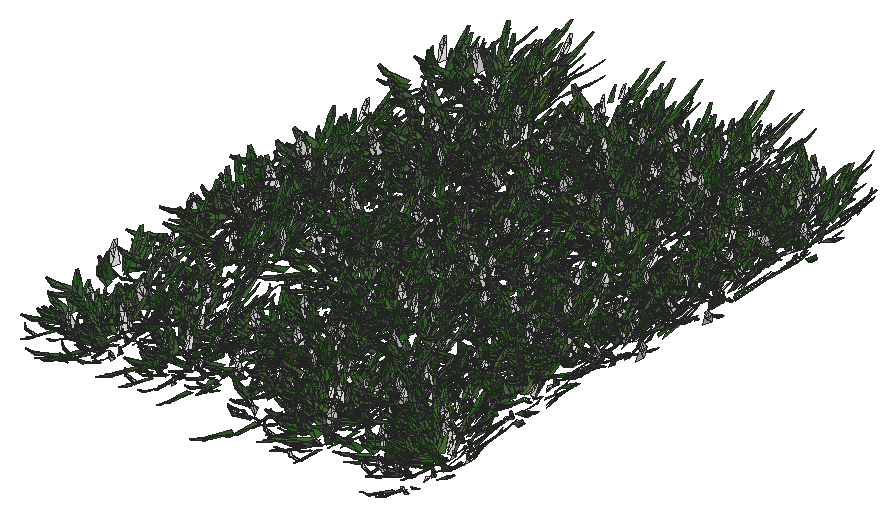
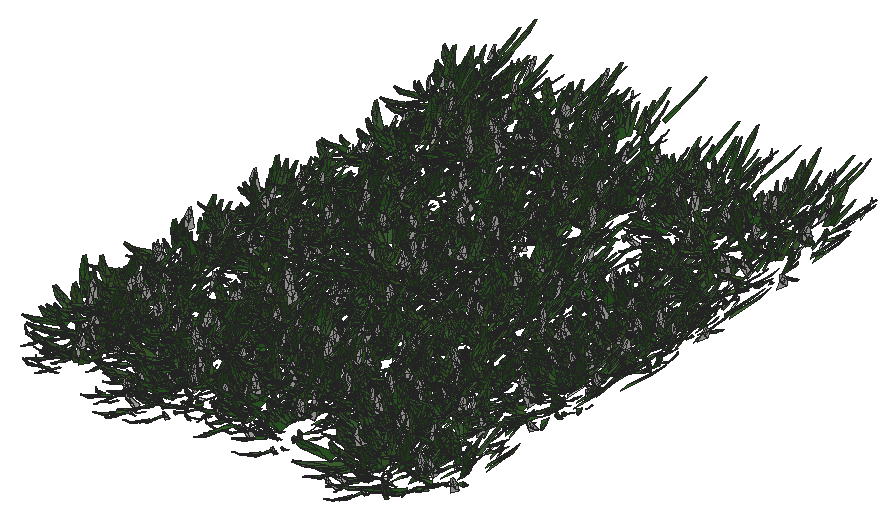
# SketchUp Ruby script. Lengths in inches.
U = 1.inch
M = Sketchup.active_model
def pt(a) = Geom::Point3d.new(a.map { |v| v * U })
def face(e, loops, mat)
  f = e.add_face(loops[0].map { |a| pt(a) })
  loops[1..].each { |l| e.add_face(l.map { |a| pt(a) }).erase! }
  f.material = f.back_material = mat if mat
  f
end
# faces: each face lists its corners as indices into pts; further lists are holes
def faces(e, pts, list, mat = nil) = list.each { |f| face(e, (f[0].is_a?(Array) ? f : [f]).map { |l| l.map { |i| pts[i] } }, mat) }
# xy, xz, yz: faces in a plane at the given z, y or x. An outline is a flat list of corners, or four numbers for a rectangle; further outlines are holes
def ring(l) = l.size == 4 ? [[l[0], l[1]], [l[2], l[1]], [l[2], l[3]], [l[0], l[3]]] : l.each_slice(2).to_a
def flat(e, list, mat, &to3) = list.each { |f| face(e, (f[0].is_a?(Array) ? f : [f]).map { |l| ring(l).map { |u, v| to3.(u, v) } }, mat) }
def xy(e, z, list, mat = nil) = flat(e, list, mat) { |x, y| [x, y, z] }
def xz(e, y, list, mat = nil) = flat(e, list, mat) { |x, z| [x, y, z] }
def yz(e, x, list, mat = nil) = flat(e, list, mat) { |y, z| [x, y, z] }
def lines(e, pts, list) = list.each { |a, b| e.add_line(pt(pts[a]), pt(pts[b])) }
# prism: a flat outline (further loops are holes) pulled along v
def prism(e, loops, v, mat = nil)
  f = face(e, loops, mat); d = Geom::Vector3d.new(v.map { |x| x * U })
  f.pushpull(f.normal.samedirection?(d) ? d.length : -d.length)
end
def box(e, o, s, mat = nil) = prism(e, [[o, [o[0] + s[0], o[1], o[2]], [o[0] + s[0], o[1] + s[1], o[2]], [o[0], o[1] + s[1], o[2]]]], [0, 0, s[2]], mat)
def at(x, y, z, deg = 0) = Geom::Transformation.translation(pt([x, y, z])) * Geom::Transformation.rotation(ORIGIN, Z_AXIS, deg.degrees)
def axes(o, x, y, z) = Geom::Transformation.new([*x, 0, *y, 0, *z, 0, *pt(o).to_a, 1])
def part(name) = M.definitions.add(name)
# library, detail: a bought-in or finely detailed component or shape, given as its bounding box
def library(name, o, s) = part(name).tap { |d| box(d.entities, o, s) }
def detail(e, o, s) = box(e.add_group.entities, o, s)
def put(e, d, t, mat = nil) = e.add_instance(d, t).tap { |i| i.material = mat if mat }
def group(e, t, mat = nil) = e.add_group.tap { |g| g.transformation = t; g.material = mat if mat }.entities
root = M.entities
M.materials.add("Material10").color = [48, 90, 38]
M.materials.add("Material11").color = [68, 110, 48]
M.materials.add("Material12").color = [48, 90, 48]
M.materials.add("Material13").color = [58, 110, 58]
M.materials.add("Material14").color = [58, 90, 38]
M.materials.add("Material15").color = [68, 100, 58]
M.materials.add("Material16").color = [48, 100, 38]
M.materials.add("Material9").color = [68, 110, 58]
c1 = part("grass00")
p = [[-0.6875,0.15,0],[-0.56,0.08,5.52],[-0.04,0.03,2.76],[0.48,-0.02,0],[0.35,-0.02,5.52],[-0.1,-0.14,5.52],
  [-0.12,0.65,8.37],[-0.42,0.65,8.37]]
faces(c1.entities,p,[[0,1,2,3],[3,2,4],[1,5,2],[5,4,2],[1,6,5],[4,5,6],[7,6,1]])
c2 = part("Group16\#1")
put(c2.entities,c1,axes([1.44,-0.61,-0.01],[0.05352,0.12609,0],[-0.10704,0.04543,0.07239],[0.06664,-0.02828,0.11628]),"Material12")
put(c2.entities,c1,axes([0.76,-0.15,-0.01],[0.04676,0.24062,0],[-0.23162,0.04501,0.06642],[0.0652,-0.01267,0.23595]),"Material9")
put(c2.entities,c1,axes([0.79,0.01,-0.01],[-0.00606,0.34651,0],[-0.34381,-0.00602,0.0432],[0.04319,0.00076,0.34386]))
put(c2.entities,c1,axes([1,0.23,-0.01],[-0.07192,0.31144,0],[-0.28722,-0.06632,0.1236],[0.12043,0.02781,0.29478]),"Material11")
put(c2.entities,c1,axes([1.66,0.77,-0.01],[-0.13828,0.29651,0],[-0.21551,-0.1005,0.22471],[0.20365,0.09498,0.23779]),"Material16")
put(c2.entities,c1,axes([0.6875,0.52,-0.01],[-0.18126,0.24051,0],[-0.22746,-0.17142,0.09788],[0.07817,0.05891,0.28481]),"Material11")
put(c2.entities,c1,axes([0.68,0.78,-0.01],[-0.215,0.18688,0],[-0.12385,-0.14248,0.21334],[0.13995,0.16101,0.18878]),"Material9")
put(c2.entities,c1,axes([0.56,1,-0.01],[-0.13756,0.07624,0],[-0.06159,-0.11112,0.0927],[0.04494,0.08108,0.12705]),"Material11")
put(c2.entities,c1,axes([0.2,0.64,-0.01],[-0.23729,0.07254,0],[-0.05711,-0.18681,0.153],[0.04473,0.14632,0.19535]),"Material16")
put(c2.entities,c1,axes([0.0625,0.72,-0.01],[-0.28874,0.02525,0],[-0.02179,-0.24916,0.14647],[0.01276,0.14591,0.25012]),"Material9")
put(c2.entities,c1,axes([-0.08,0.62,-0.01],[-0.34089,-0.04187,0],[0.03255,-0.26504,0.216],[-0.02633,0.21439,0.26703]),"Material16")
put(c2.entities,c1,axes([-0.34,0.98,-0.01],[-0.14314,-0.0493,0],[0.04397,-0.12769,0.06843],[-0.02228,0.0647,0.13505]),"Material16")
put(c2.entities,c1,axes([-0.87,1.45,-0.01],[-0.23488,-0.14114,0],[0.13761,-0.22901,0.06087],[-0.03135,0.05217,0.26717]))
put(c2.entities,c1,axes([-0.72,0.77,-0.01],[-0.14208,-0.13251,0],[0.07209,-0.0773,0.16301],[-0.11118,0.11922,0.1057]),"Material16")
put(c2.entities,c1,axes([-0.62,0.43,-0.01],[-0.14845,-0.21203,0],[0.18654,-0.13061,0.12304],[-0.10079,0.07057,0.22772]),"Material9")
put(c2.entities,c1,axes([-0.68,0.29,-0.01],[-0.13639,-0.32136,0],[0.31723,-0.13464,0.05579],[-0.05136,0.0218,0.34462]),"Material10")
put(c2.entities,c1,axes([-0.64,0.125,-0.01],[-0.0458,-0.23569,0],[0.22124,-0.043,0.08276],[-0.08124,0.01579,0.22538]),"Material13")
put(c2.entities,c1,axes([-1.6,-0.03,-0.01],[0.00576,-0.32897,0],[0.27526,0.00482,0.18018],[-0.18015,-0.00315,0.2753]),"Material11")
put(c2.entities,c1,axes([-1.36,-0.31,-0.01],[0.05718,-0.24765,0],[0.18172,0.04196,0.17267],[-0.16825,-0.03885,0.1865]),"Material16")
put(c2.entities,c1,axes([-1.54,-0.72,-0.01],[0.06537,-0.14017,0],[0.13555,0.06321,0.03939],[-0.0357,-0.01665,0.14956]))
put(c2.entities,c1,axes([-1.19,-0.9,-0.01],[0.09597,-0.12735,0],[0.11214,0.08451,0.07557],[-0.06035,-0.04548,0.14042]),"Material15")
put(c2.entities,c1,axes([-0.47,-0.54,-0.01],[0.11588,-0.10072,0],[0.0618,0.0711,0.12124],[-0.07953,-0.0915,0.0942]))
put(c2.entities,c1,axes([-0.47,-0.84,-0.01],[0.11927,-0.0661,0],[0.06603,0.11913,0.00646],[-0.00313,-0.00565,0.13621]),"Material11")
put(c2.entities,c1,axes([-0.38,-1.24,-0.01],[0.28037,-0.08571,0],[0.0618,0.20215,0.20315],[-0.05939,-0.19428,0.21139]),"Material15")
put(c2.entities,c1,axes([-0.06,-0.66,-0.01],[0.22719,-0.01987,0],[0.01247,0.14255,0.17758],[-0.01547,-0.17691,0.1431]),"Material14")
put(c2.entities,c1,axes([0.11,-0.89,-0.01],[0.14882,0.01828,0],[-0.01058,0.08611,0.12229],[0.01491,-0.12138,0.08676]),"Material12")
put(c2.entities,c1,axes([0.25,-0.72,-0.01],[0.20481,0.07053,0],[-0.06206,0.18022,0.10291],[0.03351,-0.0973,0.1906]),"Material12")
put(c2.entities,c1,axes([0.85,-1.42,-0.01],[0.16481,0.09904,0],[-0.09472,0.15762,0.05616],[0.02893,-0.04814,0.18389]),"Material11")
put(c2.entities,c1,axes([1.01,-1.09,-0.01],[0.21858,0.20385,0],[-0.17495,0.1876,0.15339],[0.10462,-0.11218,0.25652]),"Material16")
put(c2.entities,c1,axes([1.01,-0.71,-0.01],[0.08733,0.12473,0],[-0.06445,0.04512,0.13037],[0.1068,-0.07477,0.07867]),"Material12")
c3 = part("Group15\#1")
put(c3.entities,c2,at(0,0,0))
c4 = part("3darcstudiotree_grass00\#1")
put(c4.entities,c3,at(0,0,0))
put(root,c4,axes([852.99,505.65,12.99],[-1.4574,-5.63848,0],[2.95707,-3.99377,-0.05519],[0.18301,-0.24717,1.81465]))
put(root,c4,axes([868.36,504.57,12.99],[-2.38107,1.42759,0],[-0.85109,-7.41733,-0.03948],[-0.03443,-0.30004,1.58152]))
put(root,c4,axes([880.25,505.71,12.99],[-2.65306,0.75515,0],[-0.30618,-5.6208,-0.03309],[-0.01933,-0.35489,1.60704]))
put(root,c4,axes([812.43,506.21,12.99],[0.97906,6.52331,0],[-3.045,2.38799,-0.02597],[-0.10941,0.0858,1.96681]))
put(root,c4,axes([889.31,505.75,12.99],[-0.29524,7.25073,0],[-3.22684,-0.68655,-0.02425],[-0.09592,-0.02041,1.76617]))
put(root,c4,axes([815.1875,505.93,12.99],[-1.51893,5.13574,0],[-2.21828,-3.42812,-0.04556],[-0.20111,-0.3108,1.95702]))
put(root,c4,axes([864.16,506.36,12.99],[-1.28385,6.32972,0],[-3.05533,-3.23813,-0.04346],[-0.1591,-0.16862,1.86413]))
put(root,c4,axes([829.44,506.47,12.99],[-1.67508,5.71212,0],[-2.30411,-3.53058,-0.02214],[-0.07899,-0.12104,1.63462]))
put(root,c4,axes([860.26,508.67,12.99],[-0.73247,5.58304,0],[-2.39109,-1.63916,-0.04553],[-0.16619,-0.11393,1.30482]))
put(root,c4,axes([804.88,508.77,12.99],[-1.45548,4.78195,0],[-2.53134,-4.02584,-0.02835],[-0.08051,-0.12804,1.46355]))
put(root,c4,axes([836.09,511.61,12.99],[-0.59172,-6.25795,0],[3.15122,-1.55693,-0.06129],[0.18119,-0.08952,1.3376]))
put(root,c4,axes([839.96,513.6,12.99],[1.81889,-5.12817,0],[2.27845,4.22268,-0.02965],[0.0785,0.14549,1.3715]))
put(root,c4,axes([888.95,511.52,12.99],[-2.3306,2.97499,0],[-1.43535,-5.87549,-0.05669],[-0.12758,-0.52224,1.86391]))
put(root,c4,axes([829.74,514.59,12.99],[0.32741,-6.68639,0],[2.88308,0.73767,-0.04376],[0.16602,0.04248,1.51939]))
put(root,c4,axes([813.01,514.53,12.99],[-1.23373,-7.18281,0],[2.85603,-2.56327,-0.05278],[0.2168,-0.19457,1.85719]))
put(root,c4,axes([861.77,514.1,12.99],[3.25038,2.24612,0],[-0.74618,5.64218,-0.04581],[-0.05899,0.44607,1.57403]))
put(root,c4,axes([825.73,515.14,12.99],[-1.6723,-6.27142,0],[2.4813,-3.45726,-0.05337],[0.17283,-0.24081,1.5119]))
put(root,c4,axes([849.57,516.25,12.99],[2.32247,1.67856,0],[-0.87062,6.29427,-0.04459],[-0.05663,0.40941,1.66873]))
put(root,c4,axes([884.89,514.02,12.99],[-2.80487,4.80341,0],[-1.88905,-5.76384,-0.03017],[-0.07229,-0.22059,1.72726]))
put(root,c4,axes([858.34,515.21,12.99],[-1.80171,5.10925,0],[-2.01199,-3.70729,-0.02131],[-0.08871,-0.16345,1.8955]))
put(root,c4,axes([869.47,515.44,12.99],[-3.07015,3.79092,0],[-1.53263,-6.4857,-0.03525],[-0.04956,-0.20972,1.3087]))
put(root,c4,axes([881.875,516.3125,12.99],[-0.66712,7.40109,0],[-2.61738,-1.23277,-0.03296],[-0.12425,-0.05852,1.411]))
put(root,c4,axes([876.95,518.08,12.99],[-1.93115,5.31233,0],[-2.03831,-3.87174,-0.04997],[-0.15521,-0.29482,1.46822]))
put(root,c4,axes([866.54,520.83,12.99],[2.63887,0.34184,0],[-0.16224,6.54434,-0.02759],[-0.00627,0.25286,1.57942]))
put(root,c4,axes([825.33,522.77,12.99],[1.5401,-6.84309,0],[2.33222,2.74265,-0.03693],[0.16201,0.19052,1.77491]))
put(root,c4,axes([870.5,523.34,12.99],[2.02638,-5.28676,0],[2.45049,4.90784,-0.04981],[0.14007,0.28052,1.67091]))
put(root,c4,axes([813.1,521.02,12.99],[-3.22187,-0.62142,0],[0.27101,-7.34215,-0.02802],[0.0096,-0.25998,1.8014]))
put(root,c4,axes([820.1875,522.0625,12.99],[-0.711,6.35229,0],[-2.74123,-1.6032,-0.04208],[-0.16176,-0.09461,1.54007]))
put(root,c4,axes([853.02,523.4375,12.99],[1.90675,3.48333,0],[-1.62246,4.64063,-0.04441],[-0.13783,0.39422,1.772]))
put(root,c4,axes([802.73,524.59,12.99],[2.32676,5.16821,0],[-2.32007,5.45779,-0.06236],[-0.17718,0.41679,1.86199]))
put(root,c4,axes([845.72,524.27,12.99],[-2.90908,1.06809,0],[-0.47179,-6.71432,-0.04907],[-0.03117,-0.44354,1.63442]))
put(root,c4,axes([873.45,524.95,12.99],[-2.41388,2.83907,0],[-1.1343,-5.03934,-0.01759],[-0.04549,-0.2021,1.92222]))
put(root,c4,axes([880.66,527,12.99],[-2.1216,-6.3783,0],[2.389,-4.15221,-0.02],[0.06882,-0.1196,1.779]))
put(root,c4,axes([835.54,526.35,12.99],[-3.3333,-0.68172,0],[0.28526,-7.28818,-0.03473],[0.01209,-0.30896,1.7157]))
put(root,c4,axes([845.32,531.41,12.99],[2.43681,-0.70234,0],[0.39054,7.08027,-0.05027],[0.02289,0.41505,1.55905]))
put(root,c4,axes([880.5,532.96,12.99],[-0.25821,-7.75837,0],[3.42476,-0.59557,-0.05882],[0.1991,-0.03462,1.5994]))
put(root,c4,axes([849.96,530.97,12.99],[-2.90283,-0.7377,0],[0.33963,-6.98326,-0.05312],[0.02325,-0.47813,1.67036]))
put(root,c4,axes([864.83,531.24,12.99],[0.69475,7.78834,0],[-3.04078,1.41733,-0.03996],[-0.13023,0.0607,1.416]))
put(root,c4,axes([816.67,533.64,12.99],[0.37282,-6.86084,0],[2.81263,0.79861,-0.05019],[0.19607,0.05567,1.53052]))
put(root,c4,axes([887.1,532.5,12.99],[0.35558,6.56207,0],[-3.3357,0.94446,-0.03401],[-0.10285,0.02912,1.40523]))
put(root,c4,axes([805.42,536.24,12.99],[1.90294,-4.7288,0],[2.2471,4.72498,-0.05921],[0.19967,0.41984,1.91907]))
put(root,c4,axes([839.71,534.08,12.99],[-2.59691,0.5149,0],[-0.25923,-6.83164,-0.04163],[-0.01656,-0.4363,1.89396]))
put(root,c4,axes([857.34,539.39,12.99],[2.43439,3.40044,0],[-1.76464,6.60107,-0.04231],[-0.09132,0.34162,1.92144]))
put(root,c4,axes([839.84,539.8,12.99],[-1.45752,-6.19148,0],[2.71951,-3.34515,-0.04084],[0.13434,-0.16525,1.58232]))
put(root,c4,axes([860.12,539.4,12.99],[-2.51578,-4.78006,0],[1.576,-4.33412,-0.01701],[0.0629,-0.17297,1.95649]))
put(root,c4,axes([815.08,541,12.99],[2.38977,3.66494,0],[-1.62004,5.51977,-0.0468],[-0.10494,0.35754,1.60535]))
put(root,c4,axes([874.49,542.68,12.99],[1.98103,-6.08526,0],[2.65627,4.51844,-0.05496],[0.13739,0.2337,1.41537]))
put(root,c4,axes([865.81,543.64,12.99],[-3.33016,-0.57714,0],[0.25097,-7.56677,-0.05601],[0.01294,-0.39002,1.39118]))
put(root,c4,axes([846.09,544.49,12.99],[0.0746,5.9936,0],[-3.01911,0.19636,-0.02239],[-0.09931,0.00646,1.83839]))
put(root,c4,axes([850.24,544.17,12.99],[-1.58504,4.29019,0],[-2.2915,-4.42372,-0.03207],[-0.11857,-0.22889,1.99077]))
put(root,c4,axes([876.75,545.08,12.99],[-0.19204,5.84834,0],[-2.72443,-0.46745,-0.02554],[-0.1116,-0.01915,1.64241]))
put(root,c4,axes([885.38,545.98,12.99],[-0.5077,7.35912,0],[-3.20418,-1.15505,-0.03641],[-0.11745,-0.04234,1.45326]))
put(root,c4,axes([852.48,549.64,12.99],[3.15458,-0.54286,0],[0.19816,6.01692,-0.02417],[0.00906,0.27525,1.80918]))
put(root,c4,axes([870.48,548.67,12.99],[1.1771,5.17385,0],[-2.54636,3.02707,-0.03549],[-0.12211,0.14517,1.52707]))
put(root,c4,axes([816.42,550,12.99],[3.02632,-0.99105,0],[0.349,5.56861,-0.032],[0.02684,0.4283,1.99674]))
put(root,c4,axes([840.36,549.01,12.99],[-0.58462,5.91029,0],[-3.36979,-1.7417,-0.04071],[-0.12055,-0.06231,1.43871]))
put(root,c4,axes([801.35,551.99,12.99],[2.11041,6.11928,0],[-2.06545,3.7221,-0.04305],[-0.14239,0.2566,1.51958]))
put(root,c4,axes([833.23,553.14,12.99],[-1.60574,-6.2565,0],[2.52697,-3.38882,-0.03431],[0.11337,-0.15204,1.53951]))
put(root,c4,axes([876.51,551.16,12.99],[-2.25431,2.5457,0],[-1.29842,-6.00796,-0.03032],[-0.05012,-0.23192,1.50108]))
put(root,c4,axes([805.12,550.91,12.99],[-1.92848,6.00161,0],[-2.55415,-4.28843,-0.02364],[-0.08497,-0.14266,1.93862]))
put(root,c4,axes([827.79,552.36,12.99],[-3.03045,-0.65443,0],[0.27243,-6.59187,-0.03137],[0.00982,-0.23769,1.3228]))
put(root,c4,axes([812.43,554.23,12.99],[2.3353,4.92273,0],[-2.21925,5.50107,-0.03053],[-0.09029,0.22382,1.95907]))
put(root,c4,axes([850.375,552.81,12.99],[-2.24312,5.82887,0],[-2.59367,-5.2154,-0.06393],[-0.14229,-0.28613,1.40472]))
put(root,c4,axes([835.83,554.16,12.99],[1.72753,6.45956,0],[-2.20476,3.08098,-0.02868],[-0.10456,0.14612,1.51486]))
put(root,c4,axes([848.46,559.12,12.99],[-1.22805,-6.52328,0],[3.02457,-2.97521,-0.04688],[0.1596,-0.15699,1.67419]))
put(root,c4,axes([868.99,558.25,12.99],[-2.52764,0.67669,0],[-0.29962,-5.84788,-0.03745],[-0.01856,-0.36216,1.50509]))
put(root,c4,axes([828.84,559.06,12.99],[-2.12795,-3.77701,0],[2.07578,-6.11082,-0.06125],[0.1101,-0.32411,1.36064]))
put(root,c4,axes([872.72,560.9375,12.99],[3.30833,0.81692,0],[-0.37386,7.91113,-0.03307],[-0.01185,0.2508,1.59331]))
put(root,c4,axes([845.09,560.16,12.99],[-1.95649,-5.83038,0],[2.26162,-3.96557,-0.03114],[0.1185,-0.20778,1.87535]))
put(root,c4,axes([823.93,559.13,12.99],[-3.32319,-1.70739,0],[0.6152,-6.2567,-0.03373],[0.02563,-0.26063,1.33323]))
put(root,c4,axes([889.4,561.07,12.99],[-1.7474,-5.59847,0],[2.13202,-3.47712,-0.04134],[0.18201,-0.29685,1.943]))
put(root,c4,axes([882.71,560.52,12.99],[-2.64394,-4.70193,0],[2.10499,-6.18488,-0.06227],[0.11154,-0.32773,1.37168]))
put(root,c4,axes([860.16,562.42,12.99],[1.4135,-7.23952,0],[2.95986,3.0197,-0.04062],[0.14934,0.15236,1.79015]))
put(root,c4,axes([886.85,561.05,12.99],[2.07856,3.7481,0],[-2.10175,6.0903,-0.06164],[-0.11086,0.32125,1.3518]))
put(root,c4,axes([865.9,561.49,12.99],[-2.25962,-5.14073,0],[2.21805,-5.09433,-0.05331],[0.14975,-0.34394,1.71744]))
put(root,c4,axes([832.41,563.39,12.99],[1.66204,-4.39015,0],[2.41371,4.77477,-0.03846],[0.1049,0.2075,1.57923]))
put(root,c4,axes([800.16,561.98,12.99],[-2.26266,-2.51888,0],[1.23228,-5.78396,-0.03924],[0.0859,-0.40317,1.93013]))
put(root,c4,axes([807.05,562.32,12.99],[-3.24556,-2.91538,0],[1.09584,-6.37452,-0.03326],[0.04569,-0.26579,1.54402]))
put(root,c4,axes([858.6,563.05,12.99],[-3.20164,0.80461,0],[-0.27498,-5.71731,-0.04038],[-0.0204,-0.42407,1.5952]))
put(root,c4,axes([877.9,563.14,12.99],[-1.08518,6.28319,0],[-3.06147,-2.76285,-0.02576],[-0.0813,-0.07337,1.53201]))
put(root,c4,axes([852.31,563.375,12.99],[-2.65665,4.62743,0],[-1.7035,-5.11023,-0.04347],[-0.11366,-0.34096,1.66314]))
put(root,c4,axes([803.65,563.48,12.99],[-2.01396,5.33847,0],[-2.62607,-5.17661,-0.04683],[-0.13903,-0.27406,1.86493]))
put(root,c4,axes([809.43,567.39,12.99],[2.31786,-4.07708,0],[1.57903,4.69065,-0.03629],[0.08811,0.26173,1.41389]))
put(root,c4,axes([850.25,568.15,12.99],[3.37025,-0.741,0],[0.33309,7.91597,-0.06081],[0.01765,0.4194,1.44654]))
put(root,c4,axes([873.7,568.48,12.99],[1.82139,-5.98472,0],[2.10675,3.35024,-0.02795],[0.12137,0.19301,1.86246]))
put(root,c4,axes([812.13,569.21,12.99],[2.70657,0.01219,0],[-0.0049,5.68045,-0.0306],[-0.00034,0.39037,1.9022]))
put(root,c4,axes([840.26,569.43,12.99],[2.23742,2.46538,0],[-1.09622,5.19834,-0.04063],[-0.07804,0.37007,1.53169]))
put(root,c4,axes([823.875,568.59,12.99],[-3.45981,1.22272,0],[-0.39983,-5.91155,-0.03554],[-0.02778,-0.41075,1.83631]))
put(root,c4,axes([804.48,571.53,12.99],[0.52589,-5.69614,0],[3.19216,1.53995,-0.04294],[0.126,0.06079,1.34209]))
put(root,c4,axes([856.76,571.46,12.99],[-0.35187,-6.78121,0],[3.07514,-0.83377,-0.02638],[0.08909,-0.02416,1.44452]))
put(root,c4,axes([869.74,569.67,12.99],[0.65067,6.54246,0],[-3.24751,1.68762,-0.06457],[-0.19925,0.10354,1.44574]))
put(root,c4,axes([829.5,571.44,12.99],[-1.60291,-6.07943,0],[2.15074,-2.96305,-0.03107],[0.12859,-0.17716,1.66455]))
put(root,c4,axes([860.02,572.91,12.99],[1.13793,-5.04136,0],[2.78043,3.27934,-0.04957],[0.1772,0.20899,1.72633]))
put(root,c4,axes([885.14,571.39,12.99],[-2.7214,-1.55169,0],[0.64329,-5.89517,-0.04204],[0.04537,-0.41582,1.62585]))
put(root,c4,axes([814.9375,573.63,12.99],[2.65986,-1.80196,0],[0.71387,5.506,-0.03127],[0.03837,0.29597,1.48816]))
put(root,c4,axes([844.01,572.72,12.99],[1.01083,5.48152,0],[-2.89471,2.78925,-0.04214],[-0.17447,0.16812,1.93625]))
put(root,c4,axes([803.75,578.67,12.99],[1.55106,-4.40014,0],[2.61135,4.80987,-0.04335],[0.11342,0.2089,1.54559]))
put(root,c4,axes([873.3,578.83,12.99],[1.85863,-5.65045,0],[2.79417,4.8025,-0.05965],[0.1964,0.33757,1.97549]))
put(root,c4,axes([833.6875,576.82,12.99],[-2.58612,-2.20778,0],[1.17469,-7.18988,-0.03885],[0.05262,-0.32206,1.78292]))
put(root,c4,axes([877.1875,579.49,12.99],[3.08374,-0.337,0],[0.11769,5.62734,-0.03217],[0.00788,0.37663,1.73328]))
put(root,c4,axes([828.51,580.52,12.99],[0.08733,-7.9419,0],[2.89886,0.16655,-0.05528],[0.22204,0.01276,1.59813]))
put(root,c4,axes([849.59,579.93,12.99],[-1.15076,-7.02922,0],[3.20384,-2.74064,-0.05081],[0.15149,-0.12959,1.49393]))
put(root,c4,axes([845.95,581.6875,12.99],[2.16351,-3.14925,0],[1.41509,5.07972,-0.0345],[0.09485,0.34047,1.8497]))
put(root,c4,axes([885.41,579.84,12.99],[0.1113,5.63218,0],[-2.73633,0.28256,-0.0329],[-0.17342,0.01791,1.98251]))
put(root,c4,axes([890.27,581.6875,12.99],[-2.23602,-4.99913,0],[2.07036,-4.83873,-0.0483],[0.13186,-0.30816,1.58573]))
put(root,c4,axes([809.34,581.74,12.99],[-2.91102,-3.24885,0],[1.51961,-7.11461,-0.06565],[0.1031,-0.48269,1.70067]))
put(root,c4,axes([820.73,583.67,12.99],[-0.54687,-6.17378,0],[2.7682,-1.28126,-0.04711],[0.1797,-0.08317,1.50792]))
put(root,c4,axes([801.32,581.74,12.99],[-2.98379,-0.69531,0],[0.32782,-7.35077,-0.03002],[0.01098,-0.24613,1.59842]))
put(root,c4,axes([828.12,586.77,12.99],[-1.12297,-6.7513,0],[3.24762,-2.82262,-0.02869],[0.07921,-0.06884,1.40786]))
put(root,c4,axes([836.04,587.03,12.99],[-0.95373,-6.80216,0],[2.91754,-2.13748,-0.03893],[0.14493,-0.10618,1.64312]))
put(root,c4,axes([883.01,588.375,12.99],[2.8313,4.41831,0],[-1.6421,5.49838,-0.02215],[-0.05923,0.19831,1.8946]))
put(root,c4,axes([865.1,589.73,12.99],[1.78996,-5.10233,0],[2.42773,4.4502,-0.04277],[0.12531,0.22971,1.60323]))
put(root,c4,axes([803.27,589.24,12.99],[2.78821,2.27626,0],[-1.15946,7.42104,-0.02984],[-0.033,0.21122,1.55474]))
put(root,c4,axes([851.99,588.33,12.99],[-2.77583,-4.90355,0],[1.98262,-5.86445,-0.06061],[0.11968,-0.354,1.43628]))
put(root,c4,axes([820.84,589.99,12.99],[2.73638,0.13485,0],[-0.05769,6.11729,-0.0399],[-0.00442,0.46833,1.8861]))
put(root,c4,axes([841.42,590.68,12.99],[2.71897,0.8946,0],[-0.4236,6.72716,-0.04848],[-0.02557,0.40614,1.51023]))
put(root,c4,axes([888.82,590.3,12.99],[3.03645,1.93549,0],[-0.7103,5.82269,-0.03867],[-0.05028,0.41218,1.75619]))
put(root,c4,axes([860.07,591.58,12.99],[2.32563,-1.97622,0],[1.0064,6.18842,-0.02775],[0.04696,0.28874,1.92398]))
put(root,c4,axes([812.02,589.67,12.99],[-3.07362,-0.06655,0],[0.03292,-7.94545,-0.04475],[0.00127,-0.30764,1.43393]))
put(root,c4,axes([867.98,591.37,12.99],[-2.94786,3.38613,0],[-1.22018,-5.55051,-0.0516],[-0.12101,-0.55045,1.94674]))
put(root,c4,axes([843.88,591.9,12.99],[-1.50123,6.04582,0],[-2.93059,-3.80236,-0.03094],[-0.07874,-0.10216,1.35284]))
put(root,c4,axes([843.74,597.46,12.99],[2.93963,-0.43219,0],[0.216,7.67669,-0.04097],[0.00947,0.33665,1.66267]))
put(root,c4,axes([860.38,595.68,12.99],[-2.62956,-1.70091,0],[0.67288,-5.43554,-0.03071],[0.03421,-0.27638,1.38702]))
put(root,c4,axes([866,598.39,12.99],[3.24457,-1.97014,0],[0.87275,7.51027,-0.06211],[0.05478,0.47139,1.60192]))
put(root,c4,axes([822.9375,596.34,12.99],[-0.07625,6.66774,0],[-3.02885,-0.18099,-0.03889],[-0.14122,-0.00844,1.50954]))
put(root,c4,axes([821.27,598.71,12.99],[-0.23839,-5.75072,0],[3.38736,-0.73373,-0.03587],[0.12273,-0.02658,1.60406]))
put(root,c4,axes([836.24,598.65,12.99],[-2.49285,-5.43926,0],[2.26095,-5.41443,-0.04863],[0.14628,-0.35031,1.95701]))
put(root,c4,axes([853.67,597.36,12.99],[-2.9804,0.5478,0],[-0.25056,-7.12315,-0.04274],[-0.01047,-0.29752,1.31001]))
put(root,c4,axes([815.39,597.57,12.99],[-2.5937,4.97056,0],[-1.98974,-5.42522,-0.04843],[-0.10388,-0.28325,1.41858]))
put(root,c4,axes([868.73,599.66,12.99],[3.09205,3.53048,0],[-1.38455,6.33616,-0.04234],[-0.0639,0.29243,1.4356]))
put(root,c4,axes([856.2,600.94,12.99],[2.81397,-2.72741,0],[1.13396,6.11325,-0.02583],[0.04269,0.23015,1.68703]))
put(root,c4,axes([881.99,598.36,12.99],[-1.1808,6.41553,0],[-2.38617,-2.29484,-0.02216],[-0.09563,-0.09197,1.66252]))
put(root,c4,axes([847.65,601.23,12.99],[-1.94835,-5.48536,0],[2.6094,-4.84293,-0.02494],[0.08226,-0.15266,1.95866]))
put(root,c4,axes([827.9,600.88,12.99],[-1.22338,5.27333,0],[-2.21347,-2.68322,-0.02105],[-0.10183,-0.12344,1.88169]))
put(root,c4,axes([825.39,606.4,12.99],[1.55699,-6.71187,0],[3.01256,3.65161,-0.05067],[0.14506,0.17584,1.51576]))
put(root,c4,axes([839.37,604.98,12.99],[-2.63123,-4.92353,0],[1.78386,-4.98135,-0.04086],[0.1178,-0.32894,1.75811]))
put(root,c4,axes([820.36,606.5625,12.99],[1.83456,-4.46525,0],[2.03909,4.37751,-0.02466],[0.07472,0.1604,1.59511]))
put(root,c4,axes([885.32,606.97,12.99],[2.44886,-2.36198,0],[1.33512,7.23289,-0.0407],[0.05083,0.27539,1.51351]))
put(root,c4,axes([832.73,607.58,12.99],[1.94903,-6.24142,0],[2.70718,4.41731,-0.04124],[0.11484,0.18738,1.56101]))
put(root,c4,axes([888.9375,604.87,12.99],[-2.7025,0.34216,0],[-0.16171,-6.674,-0.04105],[-0.01037,-0.42804,1.83253]))
put(root,c4,axes([811.67,607.23,12.99],[0.05202,-7.34397,0],[3.47529,0.12862,-0.02796],[0.09347,0.00346,1.59394]))
put(root,c4,axes([852.65,606.07,12.99],[1.85754,4.66138,0],[-2.41325,5.02493,-0.05824],[-0.15142,0.3153,1.57486]))
put(root,c4,axes([879.04,604.92,12.99],[-1.70476,5.28626,0],[-2.10539,-3.54773,-0.0238],[-0.08539,-0.14389,1.59896]))
put(root,c4,axes([827.93,605.4,12.99],[-1.25637,6.42574,0],[-2.40386,-2.45588,-0.0353],[-0.15984,-0.16329,1.79152]))
put(root,c4,axes([866.23,607.53,12.99],[3.08918,3.63476,0],[-1.49736,6.64962,-0.04224],[-0.06825,0.30308,1.58426]))
put(root,c4,axes([881.64,609.29,12.99],[2.48701,-4.31869,0],[1.62379,4.88608,-0.03309],[0.07839,0.23589,1.44206]))
put(root,c4,axes([868.37,608.19,12.99],[-2.8365,0.59895,0],[-0.23568,-5.83204,-0.04806],[-0.01996,-0.49394,1.58689]))
put(root,c4,axes([804.93,610.5,12.99],[0.83911,-5.72905,0],[3.01878,2.31034,-0.04023],[0.11918,0.09121,1.36415]))
put(root,c4,axes([856.24,608.28,12.99],[-1.23548,5.6059,0],[-2.55924,-2.94719,-0.03585],[-0.1292,-0.14878,1.58646]))
put(root,c4,axes([816.15,610.62,12.99],[2.40191,1.83226,0],[-1.05952,7.25745,-0.04175],[-0.04378,0.29987,1.52086]))
put(root,c4,axes([836.07,610.02,12.99],[-2.59917,-0.06617,0],[0.02781,-5.70813,-0.02017],[0.00116,-0.23904,1.77597]))
put(root,c4,axes([848.28,611.02,12.99],[-2.11709,-2.7615,0],[1.34131,-5.37315,-0.04344],[0.11364,-0.45522,1.9596]))
put(root,c4,axes([862.54,614.67,12.99],[3.20276,-1.48596,0],[0.57541,6.48041,-0.04034],[0.03693,0.41591,1.82611]))
put(root,c4,axes([876.25,616.24,12.99],[0.98584,-5.86337,0],[2.61758,2.29966,-0.03841],[0.16303,0.14323,1.74904]))
put(root,c4,axes([872.29,615.91,12.99],[-0.0359,-5.71468,0],[3.37663,-0.11083,-0.06189],[0.22294,-0.00732,1.66883]))
put(root,c4,axes([889.33,617.09,12.99],[2.09933,-6.10734,0],[2.34994,4.22076,-0.04001],[0.14089,0.25305,1.83572]))
put(root,c4,axes([820.9375,617.2,12.99],[2.8259,-4.59738,0],[1.47848,4.74863,-0.02041],[0.06614,0.21244,1.95445]))
put(root,c4,axes([815.54,618.27,12.99],[1.96572,-5.92984,0],[2.27431,3.93942,-0.04967],[0.17573,0.30439,1.73743]))
put(root,c4,axes([842.23,619.46,12.99],[1.33419,-6.7568,0],[3.06424,3.16157,-0.03311],[0.12497,0.12894,1.9099]))
put(root,c4,axes([844.89,617.24,12.99],[0.659,7.41897,0],[-3.35234,1.55595,-0.02679],[-0.10083,0.0468,1.80175]))
put(root,c4,axes([880.73,618.6,12.99],[2.20218,3.72608,0],[-1.76058,5.43703,-0.05487],[-0.1166,0.36009,1.44987]))
put(root,c4,axes([864.3,618.21,12.99],[-3.306,-1.85146,0],[0.83122,-7.75547,-0.038],[0.03573,-0.33334,1.89315]))
put(root,c4,axes([885.16,617.71,12.99],[-2.2968,4.36855,0],[-2.13653,-5.86947,-0.01948],[-0.04916,-0.13506,1.80807]))
put(root,c4,axes([800.8,619.87,12.99],[2.48033,3.57038,0],[-1.49573,5.4294,-0.03908],[-0.0986,0.3579,1.82303]))
put(root,c4,axes([837.95,618.5,12.99],[-2.79217,3.56158,0],[-1.35297,-5.54231,-0.03544],[-0.07061,-0.28924,1.55733]))
put(root,c4,axes([858.3,619.6,12.99],[-0.80564,5.52606,0],[-2.3049,-1.75584,-0.02384],[-0.12278,-0.09353,1.80943]))
put(root,c4,axes([844.24,623.96,12.99],[2.19,-4.08575,0],[1.63887,4.59008,-0.03627],[0.12181,0.34117,1.88825]))
put(root,c4,axes([815.75,624.78,12.99],[3.39045,-1.28338,0],[0.56889,7.85302,-0.06031],[0.04096,0.5654,1.9859]))
put(root,c4,axes([833.51,625.08,12.99],[0.3766,-6.48144,0],[3.32393,1.00917,-0.03191],[0.11824,0.0359,1.71939]))
put(root,c4,axes([811.12,626.66,12.99],[0.76138,-6.67957,0],[2.55899,1.52414,-0.04641],[0.18239,0.10863,1.47323]))
put(root,c4,axes([851.82,624.9,12.99],[-2.64896,1.9718,0],[-0.78939,-5.54123,-0.04555],[-0.06493,-0.45576,1.60995]))
put(root,c4,axes([857.69,627.5625,12.99],[0.89392,-6.76369,0],[3.03152,2.09352,-0.03916],[0.15653,0.1081,1.81408]))
put(root,c4,axes([807.04,625.58,12.99],[-3.28395,0.31374,0],[-0.11381,-6.22452,-0.02048],[-0.00457,-0.24983,1.99696]))
put(root,c4,axes([880.84,625.77,12.99],[-1.30898,4.93953,0],[-2.94357,-4.07592,-0.05645],[-0.20251,-0.28041,1.97994]))
put(root,c4,axes([861.1,628.64,12.99],[-0.43907,-6.42546,0],[2.72068,-0.97143,-0.04759],[0.16798,-0.05998,1.34947]))
put(root,c4,axes([865.83,626.21,12.99],[-1.41721,5.62928,0],[-2.98326,-3.92442,-0.03664],[-0.08905,-0.11714,1.3241]))
